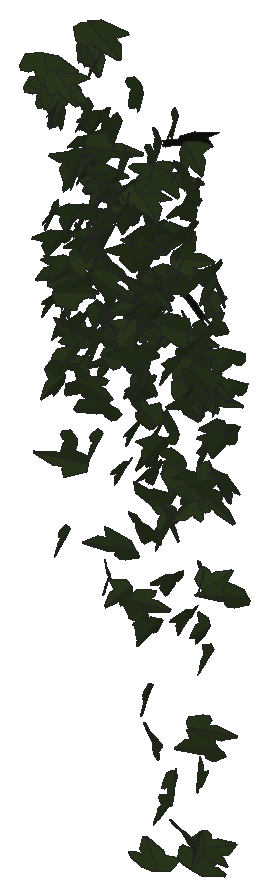
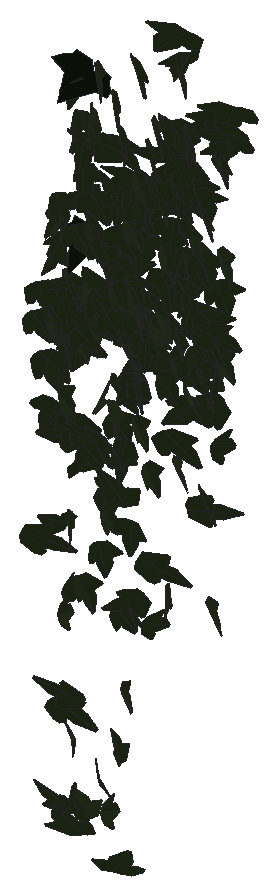
# SketchUp Ruby script. Lengths in millimetres.
U = 1.mm
M = Sketchup.active_model
def pt(a) = Geom::Point3d.new(a.map { |v| v * U })
def face(e, loops, mat)
  f = e.add_face(loops[0].map { |a| pt(a) })
  loops[1..].each { |l| e.add_face(l.map { |a| pt(a) }).erase! }
  f.material = f.back_material = mat if mat
  f
end
# faces: each face lists its corners as indices into pts; further lists are holes
def faces(e, pts, list, mat = nil) = list.each { |f| face(e, (f[0].is_a?(Array) ? f : [f]).map { |l| l.map { |i| pts[i] } }, mat) }
# xy, xz, yz: faces in a plane at the given z, y or x. An outline is a flat list of corners, or four numbers for a rectangle; further outlines are holes
def ring(l) = l.size == 4 ? [[l[0], l[1]], [l[2], l[1]], [l[2], l[3]], [l[0], l[3]]] : l.each_slice(2).to_a
def flat(e, list, mat, &to3) = list.each { |f| face(e, (f[0].is_a?(Array) ? f : [f]).map { |l| ring(l).map { |u, v| to3.(u, v) } }, mat) }
def xy(e, z, list, mat = nil) = flat(e, list, mat) { |x, y| [x, y, z] }
def xz(e, y, list, mat = nil) = flat(e, list, mat) { |x, z| [x, y, z] }
def yz(e, x, list, mat = nil) = flat(e, list, mat) { |y, z| [x, y, z] }
def lines(e, pts, list) = list.each { |a, b| e.add_line(pt(pts[a]), pt(pts[b])) }
# prism: a flat outline (further loops are holes) pulled along v
def prism(e, loops, v, mat = nil)
  f = face(e, loops, mat); d = Geom::Vector3d.new(v.map { |x| x * U })
  f.pushpull(f.normal.samedirection?(d) ? d.length : -d.length)
end
def box(e, o, s, mat = nil) = prism(e, [[o, [o[0] + s[0], o[1], o[2]], [o[0] + s[0], o[1] + s[1], o[2]], [o[0], o[1] + s[1], o[2]]]], [0, 0, s[2]], mat)
def at(x, y, z, deg = 0) = Geom::Transformation.translation(pt([x, y, z])) * Geom::Transformation.rotation(ORIGIN, Z_AXIS, deg.degrees)
def axes(o, x, y, z) = Geom::Transformation.new([*x, 0, *y, 0, *z, 0, *pt(o).to_a, 1])
def part(name) = M.definitions.add(name)
# library, detail: a bought-in or finely detailed component or shape, given as its bounding box
def library(name, o, s) = part(name).tap { |d| box(d.entities, o, s) }
def detail(e, o, s) = box(e.add_group.entities, o, s)
def put(e, d, t, mat = nil) = e.add_instance(d, t).tap { |i| i.material = mat if mat }
def group(e, t, mat = nil) = e.add_group.tap { |g| g.transformation = t; g.material = mat if mat }.entities
root = M.entities
M.materials.add("efeu1").color = [18, 25, 13]
M.materials.add("efeu2").color = [43, 57, 29]
c1 = part("ivyleaf_10")
p = [[0,12.8,-0.8],[-1.5,51.3,-10.9],[-4.9,51,-11.6],[-13.6,26.5,-7.3],[-13.2,15.9,-4.6],[-21.1,19.3,-7.2],
  [-29.5,16.3,-8.3],[-29.2,8.3,-6.2],[-19.7,-9.8,0.5],[-7.6,-13,4],[1,-12.2,5.8],[-0.4,51.1,-11.1],
  [-1.5,51.1,-10.9],[1,-12.4,5.9],[16.9,-12.4,3.5],[35.1,9.1,-5.1],[35,12.9,-6.1],[20.5,16.4,-4.9],
  [15.8,15,-3.8],[15.3,27.6,-7.1],[12.8,31.3,-7.8]]
faces(c1.entities,p,[[0,1,2,3,4,5,6,7,8,9,10],[11,12,0,13,14,15,16,17,18,19,20]],"efeu2")
c2 = part("ivyleaf_9")
p = [[39.1,54.8,31.7],[34.5,51.8,30.2],[-5.3,25.2,17.3],[-17.9,28.3,20.9],[-21.6,21.7,17],[-20.2,4.3,5.3],
  [-22.9,-0.3,2.5],[-17.1,-4,-0.6],[-2,-2.1,-1.2],[-0.7,-15.4,-10.1],[16.6,-22.3,-16.7],[21.1,-15.1,-12.5],
  [32.7,-10.7,-11],[46.1,-1.8,-6.6],[30.8,11.2,3.8]]
faces(c2.entities,p,[[0,1,2,3,4,5,6,7,8,9,10,11,12,13,14]],"efeu1")
put(root,c1,axes([1007.3,1039.5,776.9],[0.1518,-0.62324,0.17864],[0.00161,-0.17988,-0.62797],[1.23392,0.07691,-0.02116]))
put(root,c1,axes([1021.5,1050.6,815.6],[-0.52251,-0.26666,0.55039],[-0.57205,-0.46658,-0.37599],[1.0137,-0.40075,0.07152]))
put(root,c1,axes([1004.9,1030.8,1077.6],[0.4562,0.67519,0.06414],[-0.05656,0.07841,-0.71444],[-1.28957,0.23542,0.05402]))
put(root,c1,axes([1001.5,1023.8,1126.7],[1.165,0.3818,0.10176],[0.12234,0.08892,-0.72027],[-0.742,0.61412,0.04102]))
put(root,c1,axes([1009.5,1042.7,653.7],[-0.07584,-0.25558,0.66849],[0.28945,-0.65726,-0.24222],[1.33099,0.12837,0.09077]))
put(root,c1,axes([1016.8,1032.6,872.5],[-0.48716,-0.62666,0.1293],[-0.03772,-0.13143,-0.67622],[1.21719,-0.25488,0.03079]))
put(root,c1,axes([1002.7,1031.1,1089.1],[1.24631,0.27704,0.11574],[0.18939,0.06173,-0.71082],[-0.53912,0.66213,0.01785]))
put(root,c1,axes([1015.3,1041.7,787],[0.63135,-0.53622,-0.23848],[-0.08642,0.24967,-0.62455],[1.11357,0.32339,0.08674]))
put(root,c1,axes([1016,1025.1,912.6],[0.25775,-0.68489,-0.04451],[-0.00645,0.0447,-0.69813],[1.30621,0.13537,0.00533]))
put(root,c1,axes([1015.3,1048.6,424.5],[0.4454,-0.6359,0.06055],[0.04102,-0.05659,-0.67759],[1.21502,0.23502,0.00068]))
put(root,c1,axes([1016.4,1033.4,1065.7],[0.2708,-0.6955,0.01762],[0.04065,-0.01361,-0.70967],[1.32348,0.14273,0.01819]))
put(root,c1,axes([1019.2,1031.2,1058.8],[0.79915,-0.55474,-0.16486],[-0.10397,0.16478,-0.69361],[1.09649,0.41993,0.05439]))
put(root,c1,axes([1025.5,1043.7,830],[-0.58745,-0.51924,0.28521],[-0.19087,-0.27116,-0.6022],[1.1112,-0.32108,0.04734]))
put(root,c1,axes([1018.4,1035.8,742.7],[0.10843,-0.54142,-0.35837],[0.1928,0.36275,-0.53194],[1.22058,-0.0092,0.11586]))
put(root,c1,axes([1021.9,1027.3,1096.8],[1.30025,0.19789,-0.13654],[-0.2578,-0.023,-0.71111],[-0.37804,0.69632,0.01531]))
put(root,c1,axes([1047.5,1034.3,548.3],[-0.0793,-0.03002,-0.67662],[-1.19723,-0.24951,0.04981],[-0.4777,0.63032,-0.01251]))
put(root,c1,axes([1034,1046.6,910.6],[-0.46411,-0.62024,0.12857],[-0.03825,-0.13012,-0.66585],[1.20493,-0.24303,0.02838]))
put(root,c1,axes([1035.7,1037.2,572.9],[0.63991,-0.54381,-0.17276],[-0.15828,0.15167,-0.6393],[1.07435,0.34625,0.00871]))
put(root,c1,axes([1023,1044.8,789.4],[0.69978,-0.41825,0.37265],[0.53116,-0.24972,-0.55565],[0.92439,0.46011,0.03718]))
put(root,c1,axes([1027.7,1045.1,799.8],[1.22532,-0.05207,0.10376],[0.19563,-0.01602,-0.64588],[0.10268,0.65193,-0.00759]))
put(root,c1,axes([1027,1024.7,1110.6],[0.58099,0.61406,0.24078],[0.21004,0.21402,-0.68575],[-1.23761,0.32459,-0.00335]))
put(root,c1,axes([1040.3,1033.6,974.3],[0.6541,-0.60969,-0.07957],[-0.03454,0.08106,-0.69948],[1.16969,0.34334,0.02384]))
put(root,c1,axes([1027.3,1023.6,696.6],[-0.32832,-0.18034,-0.73188],[0.93447,0.54278,-0.24947],[1.08847,-0.52038,-0.00658]))
put(root,c1,axes([1037.2,1041,725],[1.06946,-0.36379,0.02764],[-0.02744,0.02857,0.66921],[-0.69382,-0.56188,0.01613]))
put(root,c1,axes([1045.2,1028.9,911.4],[0.31202,-0.6525,-0.11936],[-0.01606,0.12089,-0.67245],[1.26234,0.16282,0.02095]))
put(root,c1,axes([1043.9,1029.7,723.9],[0.69806,-0.53806,-0.0015],[-0.00406,0.00036,-0.65118],[1.02404,0.36678,-0.00156]))
put(root,c1,axes([1051.5,1035.5,992.9],[-0.88047,-0.44426,0.27239],[-0.17571,-0.2886,-0.62751],[0.9761,-0.45269,0.13274]))
put(root,c1,axes([1063.1,1035,734.2],[-0.78495,-0.14407,-0.5147],[-0.93374,-0.1559,0.43677],[-0.4036,0.64087,-0.00946]))
put(root,c1,axes([1052.8,1034.3,1004],[-0.37797,-0.65229,0.13406],[0.06822,-0.15016,-0.67754],[1.26554,-0.18672,0.07656]))
put(root,c1,axes([1054.6,1032.5,765.6],[-0.12587,-0.65872,0.04144],[0.0111,-0.04223,-0.66195],[1.2561,-0.06563,0.01]))
put(root,c1,axes([1045,1010.1,806.3],[0.0854,0.07021,0.77625],[0.19036,0.77059,-0.07548],[-1.47112,0.10379,0.03529]))
put(root,c1,axes([1060.6,1025.4,913.6],[0.2566,-0.67541,-0.14371],[-0.03744,0.14261,-0.68868],[1.31368,0.13599,0.00844]))
put(root,c1,axes([1060.2,1036,886.1],[-1.02657,0.42186,0.01176],[-0.01267,0.01057,-0.68476],[-0.8031,-0.53942,-0.00423]))
put(root,c1,axes([1049.2,1037.7,688],[-0.10843,-0.16691,-0.61965],[0.46212,-0.58145,0.1343],[-1.13056,-0.22166,0.11432]))
put(root,c1,axes([1056.7,1025.2,857],[0.01724,0.43631,0.61013],[0.03109,0.60992,-0.4364],[-1.42722,0.01856,-0.00214]))
put(root,c1,axes([1064.9,1032.6,892.1],[0.26815,-0.62519,-0.23745],[0.0088,0.24357,-0.63855],[1.27276,0.13003,0.05444]))
put(root,c1,axes([1064.3,1033,829.4],[-0.20822,-0.60226,-0.2658],[0.12689,0.25792,-0.61186],[1.24645,-0.12687,0.01789]))
put(root,c1,axes([1065.1,1033.9,1073.6],[0.52207,-0.65072,-0.08738],[-0.01261,0.09195,-0.70556],[1.2495,0.27282,0.02939]))
put(root,c1,axes([1084.6,1044.1,639.9],[-0.82808,-0.12941,0.50407],[-0.92843,-0.12743,-0.45379],[0.34498,-0.65357,-0.01133]))
put(root,c1,axes([1066.2,1038.2,1030.7],[-0.6249,-0.5543,-0.27303],[0.23319,0.24464,-0.644],[1.15262,-0.35001,-0.01773]))
put(root,c1,axes([1067.7,1028.9,1069.6],[0.16787,-0.67555,-0.229],[0.07195,0.23485,-0.67824],[1.35566,0.07119,0.06435]))
put(root,c1,axes([1069.5,1027.1,887.1],[-0.55531,-0.59657,-0.15254],[0.09702,0.14482,-0.66388],[1.16791,-0.29569,-0.01738]))
put(root,c1,axes([1072.1,1017.6,1000.6],[0.18375,-0.53787,-0.44191],[0.04693,0.44851,-0.54051],[1.32404,0.05875,0.08049]))
put(root,c1,axes([1078.1,1033.8,896.5],[-0.43947,-0.6062,0.20907],[0.02161,-0.22605,-0.64287],[1.22021,-0.21432,0.08668]))
put(root,c1,axes([1079.8,1038.9,862.2],[1.0656,-0.21536,-0.27537],[-0.3186,0.29128,-0.56818],[0.58408,0.55179,0.19246]))
put(root,c1,axes([1079.3,1020.3,738.5],[0.12599,-0.51706,-0.39918],[-0.02055,0.4003,-0.5203],[1.24303,0.05903,0.03186]))
put(root,c1,axes([1082.8,1036.1,1016.7],[0.11629,-0.67943,-0.17144],[-0.03008,0.17071,-0.68217],[1.33328,0.06311,-0.00044]))
put(root,c1,axes([1070.1,1016.8,679],[-0.78578,-0.30801,-0.48789],[0.71013,0.31507,-0.51466],[0.83759,-0.55608,-0.02137]))
put(root,c1,axes([1081.4,1033.5,595.8],[0.50131,-0.57839,0.06683],[0.04267,-0.06322,-0.63552],[1.1073,0.2643,-0.00577]))
put(root,c1,axes([1085.1,1032,1074.7],[-0.25151,-0.69695,0.09346],[-0.00202,-0.0949,-0.70918],[1.3383,-0.13112,0.01649]))
put(root,c1,axes([1080.3,1024,886.1],[0.13047,-0.55851,-0.40083],[0.29707,0.40495,-0.53754],[1.2742,-0.03722,0.16637]))
put(root,c1,axes([1079.2,1018.8,1175],[0.07956,0.72857,0.11702],[-0.01226,0.11756,-0.72966],[-1.40434,0.04025,0.013]))
put(root,c1,axes([1086.7,1024.2,1160.5],[0.39492,-0.68416,-0.15987],[-0.03889,0.16075,-0.71445],[1.3366,0.20682,0.02645]))
put(root,c1,axes([1077.8,1021.7,1175.7],[0.40031,0.70534,0.0521],[0.04298,0.04763,-0.73599],[-1.34537,0.21139,-0.00801]))
put(root,c1,axes([1084.5,1034.5,748.7],[0.18728,-0.57095,0.39731],[0.28898,-0.37396,-0.575],[1.29192,0.16641,0.07102]))
put(root,c1,axes([1092.9,1021.6,780.6],[0.27213,-0.57574,-0.30284],[-0.15345,0.292,-0.59319],[1.22855,0.164,-0.00701]))
put(root,c1,axes([1109.5,1023.4,976.5],[-0.91655,0.04123,0.55153],[-1.0471,0.03894,-0.48332],[-0.10744,-0.73116,0.00536]))
put(root,c1,axes([1077.2,1032.6,941.1],[0.54115,-0.41575,0.47022],[0.61416,-0.34593,-0.501],[1.02459,0.42695,0.05196]))
put(root,c1,axes([1091.6,1044.5,898.7],[0.06483,-0.68562,-0.00532],[-0.00574,0.00518,-0.68646],[1.30489,0.03408,-0.00276]))
put(root,c1,axes([1092.4,1029,932.9],[-0.87875,-0.52625,-0.10401],[0.13853,0.0745,-0.70007],[1.01149,-0.46739,0.00552]))
put(root,c1,axes([1102.3,1034.5,858.8],[-1.06191,0.2577,0.27413],[-0.50831,0.07405,-0.61323],[-0.50433,-0.61724,0.04088]))
put(root,c1,axes([1096.3,1031.8,973.6],[-0.20879,-0.58123,0.36956],[0.10506,-0.38043,-0.58195],[1.30665,-0.06229,0.10584]))
put(root,c1,axes([1097.6,1040.4,715.7],[-0.06125,-0.62457,0.24409],[0.04118,-0.24521,-0.62459],[1.27557,-0.02208,0.03188]))
put(root,c1,axes([1077.4,1036.7,985],[1.04391,0.17555,0.41224],[0.68733,0.21247,-0.571],[-0.50473,0.65242,0.07504]))
put(root,c1,axes([1101.8,1025.3,795.6],[0.11379,-0.2875,-0.63142],[-0.06261,0.63188,-0.29083],[1.31895,0.0548,0.04067]))
put(root,c1,axes([1121.8,1039.7,446.5],[-0.37727,-0.08508,0.65447],[-1.13843,-0.2656,-0.2157],[0.53077,-0.63015,0.00255]))
put(root,c1,axes([1103.9,1024.1,404.9],[0.23387,-0.37507,-0.55074],[-0.05337,0.55662,-0.38533],[1.26703,0.09268,0.08542]))
put(root,c1,axes([1085.9,1020,1204.2],[1.04455,0.3035,0.40505],[0.60089,0.2617,-0.62389],[-0.7529,0.62993,0.06403]))
put(root,c1,axes([1082.1,1031.4,785.2],[0.55512,-0.18018,0.59082],[1.07209,-0.19048,-0.33618],[0.48232,0.63077,0.06725]))
put(root,c1,axes([1104.3,1038.2,807.6],[0.29162,-0.55835,0.32624],[0.16216,-0.31492,-0.57899],[1.22001,0.17532,-0.00102]))
put(root,c1,axes([1108.3,1023.2,1069.6],[0.8145,-0.50023,-0.30869],[-0.10893,0.34456,-0.63771],[1.1134,0.39965,0.16343]))
put(root,c1,axes([1105.8,1044.4,791.1],[0.15585,-0.52853,0.43053],[0.15584,-0.42286,-0.53469],[1.28799,0.11512,0.0126]))
put(root,c1,axes([1112.4,1025.5,967.3],[0.36024,-0.53998,-0.39955],[-0.15859,0.39303,-0.57065],[1.26856,0.20248,0.04212]))
put(root,c1,axes([1108.8,1054.8,372.4],[-0.19416,-0.20529,0.60027],[0.12402,-0.60816,-0.19692],[1.20101,0.02961,0.11737]))
put(root,c1,axes([1111.8,1029.5,996.1],[-0.14326,-0.65296,0.24858],[0.01754,-0.25092,-0.65633],[1.3296,-0.06704,0.03544]))
put(root,c1,axes([1088.7,1022.5,1032.3],[-0.13373,-0.02384,-0.72695],[1.24383,0.31847,-0.07361],[0.60754,-0.65725,-0.0093]))
put(root,c1,axes([1113.7,1034.3,1067.9],[0.52914,-0.64417,-0.13141],[0.0241,0.1479,-0.6982],[1.251,0.26962,0.06903]))
put(root,c1,axes([1092.5,1029.3,833.1],[-0.18904,0.04464,-0.68674],[1.08389,-0.38419,-0.10734],[-0.73529,-0.57782,0.01832]))
put(root,c1,axes([1125,1045.4,954.5],[-0.83551,-0.49286,0.16997],[-0.03838,-0.20599,-0.64937],[0.99148,-0.4233,0.1181]))
put(root,c1,axes([1118.2,1035.3,952.5],[0.13362,0.57173,0.44951],[-0.07182,0.45386,-0.57136],[-1.38229,0.03168,0.07314]))
put(root,c1,axes([1099.1,1037.5,745.8],[0.19749,-0.08511,-0.7135],[1.03383,-0.46261,0.13418],[-0.89521,-0.55302,-0.00244]))
put(root,c1,axes([1131.9,1036.2,756.7],[-0.98542,0.36658,0.27419],[-0.42877,0.1563,-0.6344],[-0.75844,-0.56466,0.0024]))
put(root,c1,axes([1128,1035.3,951.8],[0.35406,-0.63952,-0.18734],[-0.09883,0.17999,-0.66603],[1.26442,0.19314,0.0004]))
put(root,c1,axes([1127.2,1033.6,573.3],[0.0577,-0.63755,0.09672],[-0.00676,-0.09699,-0.63822],[1.22725,0.02944,-0.00806]))
put(root,c1,axes([1130,1037.6,974],[-0.41289,-0.64043,-0.11482],[0.13146,0.09768,-0.67535],[1.23131,-0.22518,0.0336]))
put(root,c1,axes([1132.3,1024.5,1027],[0.48251,-0.61713,-0.25077],[-0.0776,0.25344,-0.66492],[1.2654,0.25086,0.05485]))
put(root,c1,axes([1133.7,1043.1,987.3],[0.06159,-0.68955,-0.00584],[-0.01901,0.00537,-0.69024],[1.31226,0.03244,-0.00972]))
put(root,c1,axes([1134.8,1024.7,962.8],[0.03937,-0.57405,-0.40253],[0.03249,0.403,-0.57384],[1.33397,0.00713,0.02586]))
put(root,c1,axes([1136.7,1034.2,946.7],[-0.34495,-0.6679,0.0763],[-0.01145,-0.07741,-0.6919],[1.27936,-0.18077,0.01438]))
put(root,c1,axes([1114.3,1031.9,732.9],[0.68631,0.18849,0.51579],[0.75035,0.34068,-0.40013],[-0.72755,0.52917,0.07388]))
put(root,c1,axes([1137.2,1026.2,800.1],[0.41861,-0.58813,-0.24273],[-0.08552,0.24183,-0.62666],[1.20789,0.22095,0.03976]))
put(root,c1,axes([1140.2,1040.9,697.7],[0.39212,-0.57003,-0.26053],[-0.08813,0.25965,-0.60473],[1.18956,0.20714,0.04108]))
put(root,c1,axes([1142.7,1035.9,634.6],[0.16238,-0.62946,0.06615],[0.00581,-0.06634,-0.63519],[1.20457,0.08517,-0.00585]))
put(root,c1,axes([1146.5,1032.8,781.6],[-0.60901,-0.44489,0.41652],[-0.04016,-0.46207,-0.50976],[1.15919,-0.24974,0.20117]))
put(root,c1,axes([1148,1028.5,897.3],[-1.01729,-0.51019,0.01267],[-0.01525,-0.00995,-0.73892],[0.97117,-0.53457,0.00167]))
put(root,c1,axes([1147.1,1038.6,957.9],[-0.27655,-0.67577,-0.0284],[-0.01668,0.03093,-0.69105],[1.28716,-0.14479,-0.01506]))
put(root,c1,axes([1147.4,1043.2,921.9],[0.00376,-0.66951,0.11793],[-0.00339,-0.11793,-0.66951],[1.29382,0.00164,-0.0021]))
put(root,c1,axes([1152.2,1040.1,488],[-1.03202,0.28859,0.2173],[-0.37184,0.09539,-0.61422],[-0.5783,-0.57633,0.00715]))
put(root,c1,axes([1145.4,1046.4,737.5],[0.48201,-0.67703,0.0631],[0.05191,-0.05717,-0.72283],[1.29306,0.25467,0.00549]))
put(root,c1,axes([1148.6,1036.3,813.1],[0.08849,-0.66784,-0.00346],[0.00287,0.00357,-0.66945],[1.27104,0.04648,0.00175]))
put(root,c1,axes([1150.1,1023.1,834.6],[0.47134,-0.57451,-0.26696],[-0.08503,0.27009,-0.62267],[1.20269,0.24425,0.0606]))
put(root,c1,axes([1162.8,1037,817.3],[-0.3276,-0.19334,0.64929],[-0.60951,-0.56712,-0.25377],[1.13619,-0.35998,0.05108]))
put(root,c1,axes([1150.8,1041.3,831.2],[0.63089,-0.57992,-0.07876],[-0.0591,0.07296,-0.66791],[1.11227,0.33281,0.00918]))
put(root,c1,axes([1152.7,1021.6,752.3],[-0.98666,-0.54364,-0.07649],[0.099,0.05609,-0.7512],[1.04014,-0.52102,-0.00106]))
put(root,c1,axes([1146.4,1037.1,695],[-0.44534,-0.42443,-0.45458],[0.38979,0.40601,-0.48451],[1.11762,-0.31073,-0.01216]))
put(root,c1,axes([1154.7,1024.2,789.1],[0.47679,-0.54009,-0.30576],[-0.15082,0.29919,-0.59342],[1.17152,0.25832,0.04804]))
put(root,c1,axes([1147.7,1034.1,722],[0.71669,-0.5015,0.19223],[0.21133,-0.157,-0.62712],[1.00009,0.39256,-0.00524]))
put(root,c1,axes([1154.8,1023,1137.9],[0.72289,-0.58871,-0.22389],[-0.10376,0.22974,-0.69658],[1.19423,0.37632,0.07501]))
put(root,c1,axes([1159.4,1031.1,818.8],[-1.36287,0.16899,0.1082],[-0.20019,0.02536,-0.73576],[-0.32521,-0.72378,-0.00052]))
put(root,c1,axes([1161.6,1043.8,905.5],[-0.85384,-0.45978,0.22389],[-0.16156,-0.22675,-0.63575],[0.95979,-0.4472,0.09216]))
put(root,c1,axes([1157.1,1037.2,700.6],[0.25234,-0.58806,-0.3005],[0.08572,0.31383,-0.59429],[1.25393,0.09689,0.1011]))
put(root,c1,axes([1158.3,1034.8,696.2],[-0.18993,-0.48567,-0.50798],[0.21025,0.49585,-0.49578],[1.32093,-0.14875,0.00587]))
put(root,c1,axes([1177.8,1022.9,662.3],[0.63542,-0.06081,0.61841],[-1.12803,0.17971,0.33766],[-0.35524,-0.67942,0.03396]))
put(root,c1,axes([1160.4,1037.2,598.5],[-0.08014,-0.52875,-0.38857],[0.2291,0.37654,-0.52541],[1.22763,-0.10479,0.07269]))
put(root,c1,axes([1154.4,1032,366],[0.76355,-0.42822,0.30697],[0.38004,-0.23347,-0.58667],[0.92795,0.44797,-0.01232]))
put(root,c1,axes([1148.8,1029,382.9],[-0.37439,-0.24079,-0.58709],[0.83974,0.38984,-0.30773],[0.86794,-0.48104,0.04448]))
put(root,c1,axes([1159.2,1040,249.3],[0.41586,-0.54931,0.2742],[0.26873,-0.23828,-0.58987],[1.13713,0.2572,0.03912]))
put(root,c1,axes([1186.7,1028.3,842.3],[-0.72324,0.08081,-0.59231],[-1.13763,-0.06087,0.37519],[-0.01541,0.7011,0.10085]))
put(root,c1,axes([1150.6,1030.5,982.8],[1.07668,0.29753,0.29738],[0.50238,0.13697,-0.63919],[-0.62337,0.62427,-0.00149]))
put(root,c1,axes([1171.8,1038.6,814.7],[-0.0667,-0.6328,0.20775],[-0.05095,-0.20653,-0.6336],[1.26656,-0.04163,-0.01455]))
put(root,c1,axes([1170.4,1033.3,1039.3],[0.52935,-0.56193,-0.33488],[-0.06184,0.35157,-0.61694],[1.24344,0.25671,0.11188]))
put(root,c1,axes([1170,1041.8,-2.5],[0.9588,0.37937,0.10367],[-0.16832,-0.05488,0.63058],[0.72932,-0.5114,0.00923]))
put(root,c1,axes([1161.5,1041.3,750.7],[0.63651,-0.46336,0.32616],[0.37635,-0.25949,-0.5714],[1.01064,0.38846,0.00736]))
put(root,c1,axes([1170.4,1031.8,893.8],[0.03685,-0.6638,0.17093],[0.0514,-0.17013,-0.66374],[1.30355,0.02547,0.02134]))
put(root,c1,axes([1171,1036.5,581],[-0.17068,-0.61593,-0.20414],[0.05872,0.2018,-0.62243],[1.23355,-0.09483,0.00139]))
put(root,c1,axes([1156.7,1052.7,165.8],[-0.55107,0.23475,0.54766],[0.81153,-0.34368,0.37275],[0.79211,0.51542,-0.00088]))
put(root,c1,axes([1174.5,1031.2,356.8],[-0.1981,-0.57947,0.32447],[0.00403,-0.32872,-0.58638],[1.26396,-0.08977,0.05272]))
put(root,c1,axes([1165.4,1047.5,592.7],[0.4643,-0.4976,0.40781],[0.38376,-0.35503,-0.55383],[1.16276,0.31588,0.01995]))
put(root,c1,axes([1178.2,1041.7,649.1],[0.1219,-0.60995,-0.29481],[-0.08791,0.2915,-0.61315],[1.28634,0.07772,-0.01397]))
put(root,c1,axes([1160.9,1044.4,528],[-0.96528,-0.02251,0.41112],[0.77972,0.03734,0.50747],[-0.078,0.65182,-0.01487]))
put(root,c1,axes([1178,1048.2,779.6],[-0.41743,-0.57746,0.25104],[0.0316,-0.27104,-0.60897],[1.19796,-0.19407,0.10354]))
put(root,c1,axes([1181.3,1032.9,626.1],[-0.33463,-0.55983,0.28973],[-0.02908,-0.29692,-0.58299],[1.19934,-0.1634,0.0667]))
put(root,c1,axes([1179,1026,942.7],[-0.4989,-0.60669,-0.21946],[0.12839,0.20981,-0.66059],[1.22114,-0.26993,-0.02021]))
put(root,c1,axes([1186.2,1028.7,1020.9],[1.23178,-0.06851,-0.29641],[-0.55883,0.04167,-0.65076],[0.15153,0.71064,0.00958]))
put(root,c1,axes([1176.2,1055.5,80.4],[0.11434,-0.19934,0.62727],[0.37799,-0.59503,-0.20812],[1.19427,0.20741,0.00582]))
put(root,c1,axes([1186.2,1031.2,826],[0.09071,-0.68054,-0.00545],[-0.00295,0.00536,-0.68221],[1.29525,0.04767,-0.00117]))
put(root,c1,axes([1184.7,1045.9,495.9],[0.13518,-0.52918,0.35272],[0.19432,-0.34082,-0.53189],[1.19465,0.11532,0.04661]))
put(root,c1,axes([1191.9,1018.7,1074],[0.35085,-0.48745,-0.49833],[-0.17497,0.49396,-0.51719],[1.31513,0.19576,0.06414]))
put(root,c1,axes([1191.8,1052.1,796.6],[-0.50278,-0.54315,0.26373],[0.10481,-0.30834,-0.57987],[1.14435,-0.2104,0.16898]))
put(root,c1,axes([1192.9,1043.4,877.1],[-0.59014,-0.57285,0.18808],[0.05899,-0.22636,-0.63834],[1.14599,-0.28334,0.12971]))
put(root,c1,axes([1167.3,1031.1,862.3],[0.68781,-0.22205,0.61466],[1.13065,-0.18109,-0.41472],[0.51836,0.68965,0.089]))
put(root,c1,axes([1192.5,1045.1,804.3],[-0.17019,-0.59036,0.31044],[0.07291,-0.31724,-0.59226],[1.26734,-0.06102,0.07576]))
put(root,c1,axes([1194.1,1036.1,844.5],[0.48101,-0.58427,-0.23219],[-0.09194,0.23146,-0.63502],[1.19303,0.2534,0.04467]))
put(root,c1,axes([1192.5,1041.8,521.8],[-0.22419,-0.38739,0.5028],[0.32215,-0.51204,-0.35486],[1.16427,0.06708,0.195]))
put(root,c1,axes([1182,1028.1,934],[-0.80872,0.20041,0.53617],[0.93008,-0.22066,0.46978],[0.5672,0.64757,-0.00585]))
put(root,c1,axes([1204.6,1044.7,938.6],[-0.88905,-0.42349,0.25015],[-0.18337,-0.25952,-0.61928],[0.91797,-0.46199,0.11857]))
put(root,c1,axes([1186.3,1054.6,124.6],[0.60934,-0.34602,0.48583],[0.59943,-0.37017,-0.4712],[0.964,0.44889,-0.01409]))
put(root,c1,axes([1202.2,1044.8,600.9],[0.90074,-0.42678,-0.18837],[-0.24707,0.13725,-0.63712],[0.85278,0.49055,0.01438]))
put(root,c1,axes([1189.5,1037.1,523.9],[-0.5802,0.44976,-0.37554],[0.36307,-0.32407,-0.54299],[-1.05439,-0.35908,0.01967]))
put(root,c1,axes([1199.7,1042.3,643.4],[-0.4835,0.46707,0.36591],[0.22827,-0.3494,0.52927],[1.10593,0.27632,0.05073]))
put(root,c1,axes([1204.2,1033,435.4],[-0.33919,-0.62832,-0.00984],[0.00556,0.00939,-0.6531],[1.19594,-0.17825,0.00024]))
put(root,c1,axes([1179.7,1037.4,1014.5],[0.2754,0.01205,-0.68867],[1.31087,-0.00317,0.14467],[-0.00118,-0.7037,-0.01244]))
put(root,c1,axes([1212,1048.1,580.2],[-0.44438,-0.48068,0.35286],[0.04873,-0.38668,-0.50981],[1.13381,-0.17177,0.16021]))
put(root,c1,axes([1212.2,1044.9,888.3],[0.31669,-0.66597,-0.03146],[0.0009,0.03254,-0.68639],[1.26888,0.16619,0.00834]))
put(root,c1,axes([1211.2,1028.6,1111.5],[0.38408,-0.66324,-0.19052],[0.05951,0.20709,-0.68779],[1.31198,0.18477,0.08697]))
put(root,c1,axes([1211.4,1031.8,754],[0.09683,-0.53477,0.39576],[0.08706,-0.39317,-0.53715],[1.26318,0.06809,0.00668]))
put(root,c1,axes([1218.2,1053.1,746.2],[-0.41011,-0.49068,0.35974],[-0.016,-0.3792,-0.52226],[1.15784,-0.17904,0.1202]))
put(root,c1,axes([1219.9,1028.6,1048.7],[0.05907,-0.42127,-0.58695],[-0.04098,0.58669,-0.42222],[1.37441,0.0356,0.01264]))
put(root,c1,axes([1223.4,1044,384],[-0.08464,-0.69393,0.08531],[-0.02223,-0.08473,-0.69533],[1.33045,-0.04556,-0.00619]))
put(root,c1,axes([1214.7,1054.3,792],[-0.37819,0.24647,0.58049],[0.60348,-0.48706,0.31534],[1.03751,0.37314,0.02818]))
put(root,c1,axes([1230.9,1046.7,884],[-0.63238,-0.53823,0.24946],[-0.06179,-0.26899,-0.62363],[1.12734,-0.31666,0.10575]))
put(root,c1,axes([1227.7,1021.7,889.9],[0.81794,-0.51418,-0.19524],[-0.11766,0.20104,-0.66556],[1.04013,0.42708,0.07824]))
put(root,c1,axes([1229.1,1028.3,1035.6],[0.7365,-0.45428,-0.39024],[-0.16143,0.41836,-0.57113],[1.1283,0.35639,0.17301]))
put(root,c1,axes([1229.4,1030,929.3],[0.12104,-0.62394,0.279],[0.19822,-0.26808,-0.62327],[1.28559,0.10008,0.06983]))
put(root,c1,axes([1234.7,1038.8,552],[0.26089,0.32051,-0.57748],[-0.45352,-0.52606,-0.34854],[-1.17233,0.27483,0.00632]))
put(root,c1,axes([1234.8,1025.2,960.6],[-0.25847,-0.63386,-0.24451],[0.08663,0.2403,-0.64822],[1.2901,-0.14313,-0.00546]))
put(root,c1,axes([1207.9,1029.3,802.9],[0.2022,0.00216,0.70362],[1.16298,0.35251,-0.09335],[-0.66391,0.61815,0.05077]))
put(root,c1,axes([1218.9,1039.3,57.6],[-0.65182,-0.03574,0.5351],[0.89783,-0.32207,0.28042],[0.48549,0.54763,0.19984]))
put(root,c1,axes([1236.5,1034.8,725.4],[0.22484,-0.62254,0.06343],[0.04065,-0.0605,-0.63358],[1.19026,0.11966,0.00966]))
put(root,c1,axes([1236.7,1023.1,997.1],[-0.40779,-0.60456,-0.28846],[0.20057,0.26866,-0.64134],[1.25898,-0.23862,0.00874]))
put(root,c1,axes([1259.4,1042.3,198.6],[-0.60387,-0.1209,0.5577],[-0.98191,-0.21191,-0.33946],[0.46411,-0.60564,0.00745]))
put(root,c2,axes([1232.9,1015.2,1097.7],[0.82833,0.55721,0.27797],[0.32863,0.21784,-0.70704],[-1.13864,0.46823,-0.00184]))
put(root,c2,axes([1238,1020.3,868],[1.10158,-0.16573,-0.47397],[-0.8639,0.13647,-0.60204],[0.40849,0.73555,0.00491]))
put(root,c1,axes([1221.5,1027.8,577.1],[1.00495,0.05993,-0.48248],[0.91481,0.04268,0.53135],[0.13904,-0.71399,-0.00873]))
put(root,c1,axes([1232.8,1015.2,920.1],[0.05705,0.12484,0.68277],[0.29503,0.66494,-0.12839],[-1.28763,0.15789,0.00083]))
put(root,c1,axes([1250.5,1031.1,148],[0.49982,-0.28417,0.55907],[-0.63553,0.44969,0.38543],[-1.01032,-0.42345,0.03413]))
put(root,c1,axes([1244.5,1023.9,710.5],[-0.79914,-0.51086,-0.1733],[0.20834,0.13435,-0.66128],[1.00533,-0.43393,-0.00072]))
put(root,c1,axes([1246.7,1042.5,806.4],[0.61695,-0.57791,-0.11823],[-0.08454,0.11061,-0.66245],[1.11948,0.32684,0.01513]))
put(root,c1,axes([1240.7,1025.9,779.6],[-0.42485,-0.63266,0.1545],[0.12635,0.14037,0.6707],[-1.233,0.23238,0.01549]))
put(root,c1,axes([1241.6,1022.3,1080.1],[0.15571,0.69086,0.22349],[-0.0298,0.22653,-0.69453],[-1.38161,0.07297,0.04017]))
put(root,c1,axes([1227.5,1031.2,725],[0.88025,-0.12014,0.4827],[0.88331,-0.13288,-0.47779],[0.34057,0.65517,-0.00839]))
put(root,c1,axes([1246,1045.5,368.9],[-0.06177,0.09547,0.64466],[0.36353,-0.61572,0.1008],[1.18582,0.19373,0.00268]))
put(root,c1,axes([1253.5,1030.3,602],[-0.94315,-0.45076,-0.04619],[0.0652,0.03099,-0.6699],[0.85991,-0.49674,0.00013]))
put(root,c1,axes([1250.2,1020.4,1027.2],[0.03889,-0.64359,-0.32281],[0.18006,0.32254,-0.63706],[1.35844,-0.02433,0.09368]))
put(root,c1,axes([1259.6,1042.3,779.5],[-1.03807,-0.33875,0.10108],[-0.155,-0.06043,-0.64202],[0.65471,-0.55142,0.00827]))
put(root,c1,axes([1252.7,1044.9,639.6],[0.25385,-0.60424,0.29815],[0.18299,-0.28376,-0.61808],[1.26924,0.16176,0.02948]))
put(root,c1,axes([1252.6,1032.4,65.6],[0.01187,0.41985,-0.50432],[-0.12538,-0.50139,-0.41823],[-1.24259,0.0546,0.03739]))
put(root,c1,axes([1256.8,1026.8,460],[0.37252,-0.5012,-0.38955],[-0.0225,0.4047,-0.52664],[1.20792,0.16211,0.11033]))
put(root,c1,axes([1241.4,1034.5,25.1],[1.05598,0.10246,-0.33743],[0.6303,0.06473,0.56422],[0.23059,-0.64616,0.00302]))
put(root,c1,axes([1257.1,1037.4,715.5],[0.44215,-0.59093,-0.06122],[0.03319,0.07249,-0.63353],[1.1302,0.22905,0.04256]))
put(root,c1,axes([1252.4,1047,332.7],[0.13469,-0.20673,0.62952],[0.44796,-0.58396,-0.21823],[1.1788,0.24553,0.011]))
put(root,c1,axes([1237.5,1045.8,218.7],[0.25845,-0.02568,-0.62399],[1.16649,-0.11708,0.1382],[-0.22812,-0.62777,-0.00025]))
put(root,c1,axes([1267.5,1036.1,909.7],[-0.21425,-0.67832,-0.10841],[0.03916,0.10648,-0.68759],[1.30677,-0.1144,0.00283]))
put(root,c1,axes([1267.4,1032,887.4],[0.61205,-0.59057,-0.01523],[-0.0024,0.01666,-0.67241],[1.12434,0.32152,0.00686]))
put(root,c1,axes([1270.6,1032.3,728],[0.4626,-0.60077,-0.15262],[-0.09065,0.14535,-0.648],[1.17621,0.24748,0.01009]))
put(root,c1,axes([1271.1,1042,747.7],[0.12525,-0.66166,-0.0581],[0.00404,0.0586,-0.66488],[1.26412,0.06537,0.00788]))
put(root,c1,axes([1262.2,1021.8,603],[0.03908,-0.16896,-0.72847],[0.50712,0.68257,-0.15081],[1.32981,-0.25533,0.07892]))
put(root,c1,axes([1266.6,1042.3,889.9],[-0.65272,0.57727,-0.03177],[0.0322,-0.0269,-0.67146],[-1.09986,-0.34338,-0.0008]))
put(root,c1,axes([1266.5,1033.9,861.5],[0.00071,0.65266,0.11754],[-0.04581,0.11748,-0.65222],[-1.26129,-0.0039,0.02376]))
put(root,c1,axes([1254,1023.6,754.7],[-0.85835,0.06488,-0.51754],[0.95599,-0.13028,-0.45406],[-0.26742,-0.674,0.03795]))
put(root,c1,axes([1273.2,1039.1,678.6],[-0.00796,-0.58535,0.3775],[0.09346,-0.37681,-0.58374],[1.32231,0.02311,0.04353]))
put(root,c1,axes([1250.1,1033,722],[-0.26462,-0.04039,0.69606],[1.29754,0.14078,0.14435],[-0.27793,0.69571,0.0112]))
put(root,c1,axes([1296,1051.4,430.9],[-0.23384,-0.13664,0.64471],[-0.90122,-0.43782,-0.18303],[0.87234,-0.48894,-0.01628]))
put(root,c1,axes([1256,1036.7,53.2],[0.73408,-0.16844,-0.486],[0.90793,-0.10996,0.41672],[-0.366,-0.61063,0.05902]))
put(root,c1,axes([1267.5,1025.9,448.4],[0.38561,0.20728,-0.57368],[0.59668,0.48315,0.2853],[0.99582,-0.36976,0.0512]))
put(root,c1,axes([1276,1028.4,834.1],[-0.10251,-0.47309,-0.48273],[0.32218,0.45938,-0.4691],[1.24537,-0.15779,0.08162]))
put(root,c1,axes([1286.8,1048.3,783.8],[-0.67689,-0.50179,0.23544],[-0.14876,-0.23154,-0.61156],[1.04437,-0.35821,0.06549]))
put(root,c1,axes([1287.4,1038.4,679.6],[-0.48874,-0.60586,0.22977],[-0.15447,-0.21514,-0.65798],[1.22349,-0.26918,0.00871]))
put(root,c1,axes([1279.9,1033.5,610.6],[-1.14399,0.4031,-0.03478],[0.05294,-0.02096,-0.72373],[-0.7682,-0.60173,0.00192]))
put(root,c1,axes([1287.9,1032.8,670.3],[-0.54597,-0.57109,0.16216],[-0.07207,-0.16213,-0.63798],[1.12757,-0.28689,0.03774]))
put(root,c1,axes([1276.8,1040.5,733.2],[0.31699,-0.4443,0.52296],[0.45835,-0.46607,-0.47267],[1.22293,0.28985,0.0416]))
put(root,c1,axes([1262.7,1031.9,574.7],[0.54405,-0.08671,0.58241],[1.10216,-0.07576,-0.29552],[0.2028,0.64434,0.04363]))
put(root,c1,axes([1293.2,1048.8,740.3],[-0.50333,-0.53912,0.25266],[-0.11005,-0.2519,-0.59802],[1.12778,-0.26519,0.05441]))
